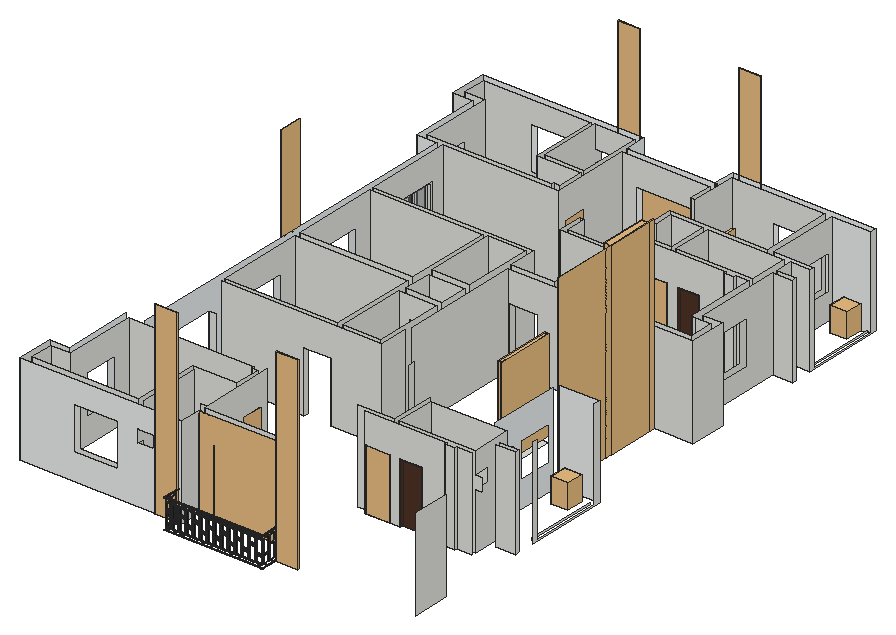
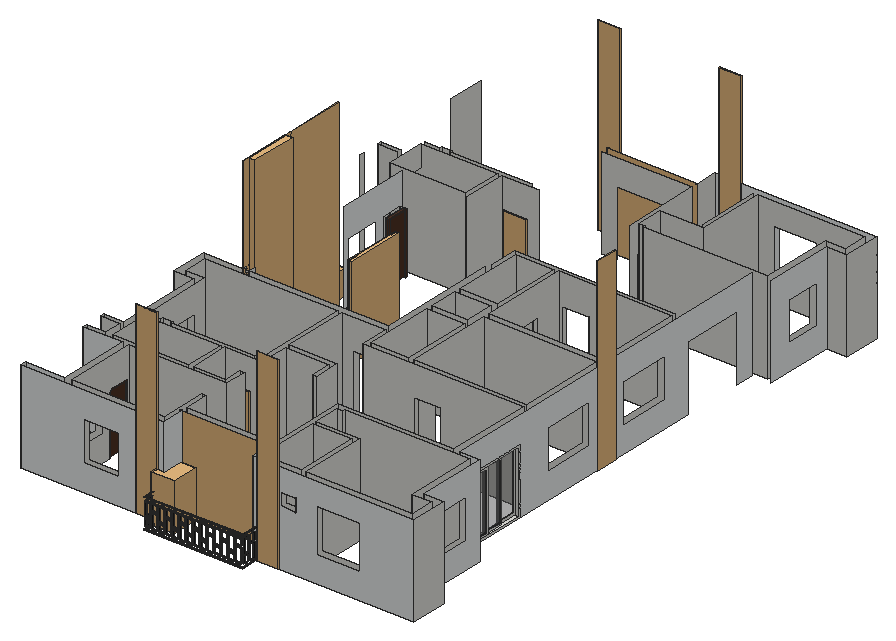
# SketchUp Ruby script. Lengths in inches.
U = 1.inch
M = Sketchup.active_model
def pt(a) = Geom::Point3d.new(a.map { |v| v * U })
def face(e, loops, mat)
  f = e.add_face(loops[0].map { |a| pt(a) })
  loops[1..].each { |l| e.add_face(l.map { |a| pt(a) }).erase! }
  f.material = f.back_material = mat if mat
  f
end
# faces: each face lists its corners as indices into pts; further lists are holes
def faces(e, pts, list, mat = nil) = list.each { |f| face(e, (f[0].is_a?(Array) ? f : [f]).map { |l| l.map { |i| pts[i] } }, mat) }
# xy, xz, yz: faces in a plane at the given z, y or x. An outline is a flat list of corners, or four numbers for a rectangle; further outlines are holes
def ring(l) = l.size == 4 ? [[l[0], l[1]], [l[2], l[1]], [l[2], l[3]], [l[0], l[3]]] : l.each_slice(2).to_a
def flat(e, list, mat, &to3) = list.each { |f| face(e, (f[0].is_a?(Array) ? f : [f]).map { |l| ring(l).map { |u, v| to3.(u, v) } }, mat) }
def xy(e, z, list, mat = nil) = flat(e, list, mat) { |x, y| [x, y, z] }
def xz(e, y, list, mat = nil) = flat(e, list, mat) { |x, z| [x, y, z] }
def yz(e, x, list, mat = nil) = flat(e, list, mat) { |y, z| [x, y, z] }
def lines(e, pts, list) = list.each { |a, b| e.add_line(pt(pts[a]), pt(pts[b])) }
# prism: a flat outline (further loops are holes) pulled along v
def prism(e, loops, v, mat = nil)
  f = face(e, loops, mat); d = Geom::Vector3d.new(v.map { |x| x * U })
  f.pushpull(f.normal.samedirection?(d) ? d.length : -d.length)
end
def box(e, o, s, mat = nil) = prism(e, [[o, [o[0] + s[0], o[1], o[2]], [o[0] + s[0], o[1] + s[1], o[2]], [o[0], o[1] + s[1], o[2]]]], [0, 0, s[2]], mat)
def at(x, y, z, deg = 0) = Geom::Transformation.translation(pt([x, y, z])) * Geom::Transformation.rotation(ORIGIN, Z_AXIS, deg.degrees)
def axes(o, x, y, z) = Geom::Transformation.new([*x, 0, *y, 0, *z, 0, *pt(o).to_a, 1])
def part(name) = M.definitions.add(name)
# library, detail: a bought-in or finely detailed component or shape, given as its bounding box
def library(name, o, s) = part(name).tap { |d| box(d.entities, o, s) }
def detail(e, o, s) = box(e.add_group.entities, o, s)
def put(e, d, t, mat = nil) = e.add_instance(d, t).tap { |i| i.material = mat if mat }
def group(e, t, mat = nil) = e.add_group.tap { |g| g.transformation = t; g.material = mat if mat }.entities
root = M.entities
M.materials.add("Polis06_194").color = [79, 50, 36]
M.materials.add("[3P0081_White-City]").color = [235, 238, 238]
M.materials.add("[Color M00]").color = [255, 255, 255]
M.materials.add("[Color M08]").color = [30, 30, 30]
M.materials.add("[Translucent Glass Gray]").color = [128, 128, 128]
M.materials["[Translucent Glass Gray]"].alpha = 0.5
c1 = part("구성 요소\#2")
prism(c1.entities,[[[0,0,0],[118.11,0,0],[118.11,0,78.74],[0,0,78.74]],[[116.14,0,76.77],[116.14,0,1.97],[1.97,0,1.97],[1.97,0,76.77]]],[0,7.875,0])
c2 = part("구성 요소\#1")
xy(c2.entities,0,[[[0,0,40.16,74.8],[2.375,2.375,37.78,72.43]]])
xy(c2.entities,1.18,[[2.375,2.375,37.78,72.43]],"[Translucent Glass Gray]")
xy(c2.entities,2.36,[[[0,0,40.16,74.8],[2.375,2.375,37.78,72.43]]])
xz(c2.entities,0,[[0,0,40.16,2.36]],"[Color M00]")
xz(c2.entities,2.375,[[2.375,0,37.78,1.18],[2.375,1.18,37.78,2.36]])
xz(c2.entities,72.43,[[2.375,0,37.78,1.18],[2.375,1.18,37.78,2.36]])
xz(c2.entities,74.8,[[0,0,40.16,2.36]],"[Color M00]")
yz(c2.entities,0,[[0,0,74.8,2.36]])
yz(c2.entities,2.375,[[2.375,0,72.43,1.18],[2.375,1.18,72.43,2.36]])
yz(c2.entities,37.78,[[2.375,0,72.43,1.18],[2.375,1.18,72.43,2.36]])
yz(c2.entities,40.16,[[0,0,74.8,2.36]])
c3 = part("구성 요소\#3")
xy(c3.entities,0,[[0,0,40.16,2.36]],"[Color M00]")
xy(c3.entities,2.375,[[2.375,0,37.78,1.18],[2.375,1.18,37.78,2.36]])
xy(c3.entities,35.83,[[38.48,0,39.47,0.39]])
xy(c3.entities,35.83,[[38.48,1.97,39.47,2.36]],"[Color M00]")
xy(c3.entities,38.98,[[38.48,0,39.47,0.39]])
xy(c3.entities,38.98,[[38.48,1.97,39.47,2.36]],"[Color M00]")
xy(c3.entities,72.43,[[2.375,0,37.78,1.18],[2.375,1.18,37.78,2.36]])
xy(c3.entities,74.8,[[0,0,40.16,2.36]],"[Color M00]")
xz(c3.entities,0,[[[0,0,40.16,74.8],[2.375,2.375,37.78,72.43],[38.48,35.83,39.47,38.98]]])
xz(c3.entities,0.39,[[38.48,35.83,39.47,38.98]])
xz(c3.entities,1.18,[[2.375,2.375,37.78,72.43]],"[Translucent Glass Gray]")
xz(c3.entities,1.97,[[38.48,35.83,39.47,38.98]],"[Color M00]")
xz(c3.entities,2.36,[[[0,0,40.16,74.8],[2.375,2.375,37.78,72.43],[38.48,35.83,39.47,38.98]]])
yz(c3.entities,0,[[0,0,2.36,74.8]])
yz(c3.entities,2.375,[[0,2.375,1.18,72.43],[1.18,2.375,2.36,72.43]])
yz(c3.entities,37.78,[[0,2.375,1.18,72.43],[1.18,2.375,2.36,72.43]])
yz(c3.entities,38.48,[[0,35.83,0.39,38.98]])
yz(c3.entities,38.48,[[1.97,35.83,2.36,38.98]],"[Color M00]")
yz(c3.entities,39.47,[[0,35.83,0.39,38.98]])
yz(c3.entities,39.47,[[1.97,35.83,2.36,38.98]],"[Color M00]")
yz(c3.entities,40.16,[[0,0,2.36,74.8]])
c4 = part("구성 요소\#4")
put(c4.entities,c2,axes([37.78,4.72,0],[1,0,0],[0,0,1],[0,-1,0]))
put(c4.entities,c3,at(75.5625,0,0))
put(c4.entities,c2,axes([0,7.09,0],[1,0,0],[0,0,1],[0,-1,0]))
c5 = part("그룹\#1")
put(c5.entities,c1,axes([0,0,0],[1.04,0,0],[0,1,0],[0,0,1]))
put(c5.entities,c4,axes([1.97,0.39,1.97],[1.02677,0,0],[0,1,0],[0,0,1]))
c6 = part("sliding door")
put(c6.entities,c5,at(0,0,0))
c7 = part("Flush door")
xy(c7.entities,0,[[0,0,4.72,1.18],[0,34.25,4.72,35.43]],"Polis06_194")
xy(c7.entities,85.26,[[0,1.18,4.72,34.25]],"Polis06_194")
xy(c7.entities,86.61,[[0,0,4.72,35.43]],"Polis06_194")
xz(c7.entities,0,[[0,0,4.72,86.61]],"Polis06_194")
xz(c7.entities,1.18,[[0,0,2.36,85.26],[2.36,0,4.72,85.26]],"Polis06_194")
xz(c7.entities,34.25,[[0,0,4.72,85.26]],"Polis06_194")
xz(c7.entities,35.43,[[0,0,4.72,86.61]],"Polis06_194")
yz(c7.entities,0,[[0,0,1.18,86.61],[34.25,0,35.43,86.61],[1.18,85.26,34.25,86.61]],"Polis06_194")
yz(c7.entities,2.36,[[1.18,0,34.25,0,34.25,85.21,1.18,85.26]],"Polis06_194")
yz(c7.entities,4.72,[[0,0,1.18,86.61],[34.25,0,35.43,86.61],[1.18,85.26,34.25,86.61]],"Polis06_194")
c8 = library("Plante 4",[-1.67,-6.5,0],[37.31,31.95,64.42])
c9 = library("Group\#241",[0,-0.25,0],[124.5,0.25,126])
c10 = library("19",[0,-1,0],[30,1,258])
c11 = library("Group\#100",[-9,0,0],[10,64,258])
c12 = library("Group\#105",[0,0,0],[0.75,82,258])
c13 = library("PINTU 6 YA",[0,-0.6875,0],[35.83,8.07,80.71])
c14 = library("Group\#2",[0,-3.15,0.41],[58,18.09,114.05])
c15 = part("Group\#70")
prism(c15.entities,[[[4.13,0,3.9375],[7.875,0,3.9375],[7.875,0,13.78],[4.13,0,13.78],[4.13,0,15.75],[7.875,0,15.75],[7.875,0,35.43],[4.13,0,35.43],[4.13,0,39.37],[3.74,0,39.37],[3.74,0,35.43],[0,0,35.43],[0,0,15.75],[3.74,0,15.75],[3.74,0,13.78],[0,0,13.78],[0,0,3.9375],[3.74,0,3.9375],[3.74,0,0],[4.13,0,0]],[[0.39,0,16.14],[0.39,0,35.04],[7.48,0,35.04],[7.48,0,16.14]],[[7.48,0,4.33],[0.39,0,4.33],[0.39,0,13.39],[7.48,0,13.39]]],[0,0.39,0],"[Color M08]")
c16 = part("Group\#69")
prism(c16.entities,[[[3.74,0,35.43],[0,0,35.43],[0,0,25.59],[3.74,0,25.59],[3.74,0,23.62],[0,0,23.62],[0,0,3.9375],[3.74,0,3.9375],[3.74,0,0],[4.13,0,0],[4.13,0,3.9375],[7.875,0,3.9375],[7.875,0,23.62],[4.13,0,23.62],[4.13,0,25.59],[7.875,0,25.59],[7.875,0,35.43],[4.13,0,35.43],[4.13,0,39.37],[3.74,0,39.37]],[[7.48,0,23.23],[7.48,0,4.33],[0.39,0,4.33],[0.39,0,23.23]],[[0.39,0,35.04],[7.48,0,35.04],[7.48,0,25.98],[0.39,0,25.98]]],[0,0.39,0],"[Color M08]")
c17 = part("Group\#71")
put(c17.entities,c15,at(0,0,0))
put(c17.entities,c16,at(9.84,0,0))
c18 = part("Group\#81")
g1 = group(c18.entities,at(0,0,0))
prism(g1,[[[24,-19.7,0],[0,-19.7,0],[0,120.08,0],[24,120.08,0],[24,118.11,0],[1.97,118.11,0],[1.97,-17.76,0],[24,-17.76,0]]],[0,0,0.79],"[Color M08]")
put(c18.entities,c17,axes([0.79,40.35,0.79],[0,1,0],[1,0,0],[0,0,1]))
put(c18.entities,c17,at(2.95,118.9,0.79))
put(c18.entities,c17,axes([0.79,79.72,0.79],[0,1,0],[1,0,0],[0,0,1]))
put(c18.entities,c17,axes([0.79,60.04,0.79],[0,1,0],[1,0,0],[0,0,1]))
put(c18.entities,c17,axes([0.79,99.41,0.79],[0,1,0],[1,0,0],[0,0,1]))
put(c18.entities,c17,axes([0.79,0.98,0.79],[0,1,0],[1,0,0],[0,0,1]))
g2 = group(c18.entities,at(0,0,40.16))
prism(g2,[[[24,-19.7,0],[0,-19.7,0],[0,120.08,0],[24,120.08,0],[24,118.11,0],[1.97,118.11,0],[1.97,-17.76,0],[24,-17.76,0]]],[0,0,0.79],"[Color M08]")
put(c18.entities,c17,axes([0.79,20.67,0.79],[0,1,0],[1,0,0],[0,0,1]))
put(c18.entities,c17,axes([0.79,-18.7,0.79],[0,1,0],[1,0,0],[0,0,1]))
put(c18.entities,c17,axes([2.95,-18.49,0.79],[1,0,0],[0,-1,0],[0,0,1]))
c19 = library("Gruppo\#3",[0,0,0],[23.62,24.19,33.46])
c20 = library("Group\#126",[0,0,0],[0.75,82,258])
xy(root,132,[[308,361.97,325.5,362.97],[198,614.97,198,656.97,207,656.97,207,630.97,321,630.97,321,624.97,207,624.97,207,614.97],[198,656.97,202,724.97],[202,656.97,203,724.97],[203,656.97,207,724.97],
  [553.5,675.97,562.5,741.97],[198,724.97,207,726.97],[384.75,779.97,402.25,783.97],[198,785.97,202,853.97],[202,785.97,203,853.97],
  [203,785.97,207,853.97],[171,1029.97,180,1031.97]])
xz(root,357.97,[[[144,132,366,258],[218,168,278,228],[306,210,327.5,228]]],"[3P0081_White-City]")
xz(root,366.97,[[[153,132,300,258],[218,168,278,228]]])
xz(root,387.97,[[366,132,386.25,132,386.25,222,470.25,222,470.25,132,490.5,132,490.5,258,366,258]],"[3P0081_White-City]")
xz(root,396.97,[[366,132,366,258,490.5,258,490.5,132,470.25,132,470.25,222,386.25,222,386.25,132]])
xz(root,399.97,[[153,132,180,258]])
xz(root,408.97,[[144,132,171,258]])
xz(root,459.97,[[300,132,300,258,360,258,360,132,333,132,333,216,309,216,309,132]])
xz(root,462.97,[[360,132,366,216]])
xz(root,495.97,[[352,132,360,258],[617.5,132,631.5,258]])
xz(root,498.97,[[180,132,352,258],[504.5,132,507,132,507,216,539,216,539,132,553.5,132,553.5,216,583.5,216,583.5,132,617.5,132,617.5,258,504.5,258],[631.5,132,652.5,258]])
xz(root,504.97,[[490.5,132,490.5,258,541.5,258,541.5,132,539,132,539,216,507,216,507,132],[547.5,132,547.5,258,652.5,258,652.5,228,661.5,228,661.5,210,652.5,210,652.5,132,583.5,132,583.5,216,553.5,216,553.5,132]])
xz(root,529,[[661.5,132,688.5,258]])
xz(root,535,[[661.5,132,688.5,258]])
xz(root,558.97,[[547.5,132,652.5,258]])
xz(root,567.97,[[622.5,132,631.5,216]])
xz(root,614.97,[[198,132,207,222]])
xz(root,624.97,[[207,132,321,132,321,216,357,216,357,132,427.5,132,427.5,258,207,258]])
xz(root,630.97,[[207,132,207,258,363,258,363,132,357,132,357,216,321,216,321,132],[369,132,421.5,258]])
xz(root,666.97,[[363,132,369,216]])
xz(root,672.97,[[631.5,132,688.5,258]],"[3P0081_White-City]")
xz(root,726.97,[[[369,132,421.5,258],[382.75,210,404.25,228]]])
xz(root,735.97,[[[372,132,421.5,258],[382.75,210,404.25,228]]])
xz(root,750.97,[[207,132,363,258]])
xz(root,759.97,[[207,132,363,258]])
xz(root,774.97,[[[372,132,421.5,258],[382.75,210,404.25,228]]])
xz(root,783.97,[[[369,132,421.5,258],[382.75,210,404.25,228]]])
xz(root,827.97,[[622.5,132,631.5,258]])
xz(root,837.97,[[430.5,132,433.5,132,433.5,216,472.5,216,472.5,132,622.5,132,622.5,258,430.5,258],[631.5,132,685.5,258]])
xz(root,846.97,[[427.5,132,427.5,258,487.5,258,487.5,132,472.5,132,472.5,216,433.5,216,433.5,132],[493.5,132,676.5,258]])
xz(root,879.97,[[207,132,321,132,321,216,357,216,357,132,363,132,363,258,207,258],[369,132,421.5,258],[649.5,132,654.5,258],[654.5,132,676.5,258]])
xz(root,885.97,[[207,132,207,258,427.5,258,427.5,132,357,132,357,216,321,216,321,132]])
xz(root,888.97,[[658.5,132,685.5,258]])
xz(root,938.47,[[421.5,132,487.5,258]])
xz(root,944.47,[[427.5,132,487.5,258]])
xz(root,972.97,[[421.5,132,427.5,258]])
xz(root,975.97,[[493.5,132,501.5,258],[617.5,132,631.5,258]])
xz(root,978.97,[[501.5,132,504,132,504,216,536,216,536,132,550.5,132,550.5,216,580.5,216,580.5,132,617.5,132,617.5,258,501.5,258],[631.5,132,649.5,258]])
xz(root,984.97,[[487.5,132,487.5,258,538.5,258,538.5,132,536,132,536,216,504,216,504,132],[544.5,132,544.5,258,649.5,258,649.5,132,580.5,132,580.5,216,550.5,216,550.5,132]])
xz(root,987.97,[[198,132,207,222]])
xz(root,1005.97,[[207,132,366,258]])
xz(root,1005.97,[[171,132,198,258]],"[3P0081_White-City]")
xz(root,1009,[[658.5,132,685.5,258]])
xz(root,1011.97,[[180,132,352,258]])
xz(root,1014.97,[[352,132,360,258],[487.5,132,493.5,258]])
xz(root,1015,[[658.5,132,685.5,258]])
xz(root,1017.47,[[360,132,366,216]])
xz(root,1038.97,[[493.5,132,538.5,258],[544.5,132,649.5,132,649.5,210,658.5,210,658.5,132,685.5,132,685.5,258,658.5,258,658.5,228,649.5,228,649.5,258,544.5,258]])
xz(root,1044.97,[[487.5,132,622.5,258]])
xz(root,1044.97,[[631.5,132,631.5,258,685.5,258,685.5,134,679.5,134,679.5,132]],"[3P0081_White-City]")
xz(root,1050.97,[[300,132,309,132,309,216,333,216,333,132,360,132,360,258,300,258]])
xz(root,1056.97,[[306,132,306,258,360,258,360,132,333,132,333,216,309,216,309,132]])
xz(root,1080.97,[[487.5,132,513.5,132,513.5,168,493.5,168,493.5,258,487.5,258]])
xz(root,1086.97,[[493.5,132,513.5,168]])
xz(root,1101.97,[[144,132,171,258]])
xz(root,1110.97,[[153,132,180,258]])
xz(root,1113.97,[[366,132,386.25,132,386.25,222,470.25,222,470.25,132,487.5,132,487.5,258,366,258]])
xz(root,1122.97,[[366,132,366,258,487.5,258,487.5,132,470.25,132,470.25,222,386.25,222,386.25,132]],"[3P0081_White-City]")
xz(root,1143.97,[[[153,132,300,258],[218,168,278,228]],[306,132,360,132,360,258,306,258,306,228,327.5,228,327.5,210,306,210],[[493.5,132,622.5,258],[550.5,168,598.5,222]]])
xz(root,1143.97,[[631.5,132,679.5,132,679.5,134,685.5,134,685.5,258,631.5,258]],"[3P0081_White-City]")
xz(root,1152.97,[[[144,132,366,258],[218,168,278,228],[306,210,327.5,228]],[[487.5,132,685.5,258],[550.5,168,598.5,222]]],"[3P0081_White-City]")
yz(root,144,[[357.97,132,408.97,258],[1101.97,132,1152.97,258]])
yz(root,153,[[366.97,132,399.97,258],[1110.97,132,1143.97,258]])
yz(root,171,[[[408.97,132,504.97,258],[426.87,168,474.87,222]],[[1005.97,132,1101.97,258],[1029.97,168,1077.97,222]]],"[3P0081_White-City]")
yz(root,180,[[[399.97,132,498.97,258],[426.87,168,474.87,222]],[[1011.97,132,1110.97,258],[1029.97,168,1077.97,222]]])
yz(root,198,[[[504.97,132,504.97,258,1005.97,258,1005.97,132,987.97,132,987.97,222,903.97,222,903.97,132,614.97,132,614.97,222,530.97,222,530.97,132],[654.97,168,726.97,222],[783.97,168,855.97,222]]],"[3P0081_White-City]")
yz(root,207,[[[630.97,132,750.97,258],[654.97,168,726.97,222]],[[759.97,132,879.97,258],[783.97,168,855.97,222]],[885.97,132,903.97,132,903.97,222,987.97,222,987.97,132,1005.97,132,1005.97,258,885.97,258]])
yz(root,300,[[366.97,132,459.97,258],[1050.97,132,1143.97,258]])
yz(root,306,[[366.97,132,453.97,132,453.97,258,366.97,258,366.97,228,357.97,228,357.97,210,366.97,210],[1056.97,132,1143.97,132,1143.97,210,1152.97,210,1152.97,228,1143.97,228,1143.97,258,1056.97,258]])
yz(root,309,[[1050.97,132,1056.97,216]])
yz(root,321,[[624.97,132,630.97,216]])
yz(root,333,[[1050.97,132,1056.97,216]])
yz(root,352,[[495.97,132,498.97,258],[1011.97,132,1014.97,258]])
yz(root,357,[[624.97,132,630.97,216],[879.97,132,885.97,216]])
yz(root,360,[[459.97,132,459.97,258,495.97,258,495.97,132,492.97,132,492.97,216,462.97,216,462.97,132],[1014.97,132,1014.97,258,1050.97,258,1050.97,132,1047.47,132,1047.47,216,1017.47,216,1017.47,132],[1056.97,132,1143.97,258]])
yz(root,363,[[630.97,132,630.97,258,750.97,258,750.97,132,690.97,132,690.97,216,666.97,216,666.97,132],[759.97,132,759.97,258,879.97,258,879.97,132,843.97,132,843.97,216,819.97,216,819.97,132]])
yz(root,366,[[357.97,132,387.97,258],[396.97,132,462.97,132,462.97,216,492.97,216,492.97,132,504.97,132,504.97,258,396.97,258],[1005.97,132,1017.47,132,1017.47,216,1047.47,216,1047.47,132,1113.97,132,1113.97,258,1005.97,258]])
yz(root,366,[[1122.97,132,1152.97,258]],"[3P0081_White-City]")
yz(root,369,[[630.97,132,666.97,132,666.97,216,690.97,216,690.97,132,726.97,132,726.97,258,630.97,258],[783.97,132,819.97,132,819.97,216,843.97,216,843.97,132,879.97,132,879.97,258,783.97,258]])
yz(root,372,[[735.97,132,774.97,258]])
yz(root,386.25,[[387.97,132,396.97,222]])
yz(root,421.5,[[630.97,132,726.97,258],[735.97,132,774.97,258],[783.97,132,879.97,258],[938.47,132,972.97,258]])
yz(root,427.5,[[624.97,132,663.97,258],[846.97,132,885.97,258],[944.47,132,972.97,258]])
yz(root,430.5,[[672.97,132,837.97,258]])
yz(root,433.5,[[663.97,132,672.97,216],[837.97,132,846.97,216]])
yz(root,487.5,[[846.97,132,938.47,258],[944.47,132,984.97,258],[1014.97,132,1044.97,258],[1080.97,132,1113.97,258]])
yz(root,487.5,[[1122.97,132,1152.97,258]],"[3P0081_White-City]")
yz(root,493.5,[[846.97,132,975.97,258],[1014.97,132,1038.97,258],[1086.97,132,1143.97,132,1143.97,258,1080.97,258,1080.97,168,1086.97,168]])
yz(root,501.5,[[975.97,132,978.97,258]])
yz(root,538.5,[[984.97,132,1038.97,258]])
yz(root,539,[[498.97,132,504.97,216]])
yz(root,541.5,[[504.97,132,564.97,258]])
yz(root,544.5,[[984.97,132,1038.97,258]])
yz(root,547.5,[[504.97,132,558.97,258]])
yz(root,553.5,[[498.97,132,504.97,216],[672.97,132,672.97,258,678.97,258,678.97,134,738.97,134,738.97,258,753.97,258,753.97,132]])
yz(root,580.5,[[978.97,132,984.97,216]])
yz(root,617.5,[[495.97,132,498.97,258],[975.97,132,978.97,258]])
yz(root,622.5,[[827.97,132,837.97,258],[[1044.97,132,1044.97,258,1143.97,258,1143.97,132,1077.97,132,1077.97,216,1047.97,216,1047.97,132],[1089.97,168,1137.97,216]]])
yz(root,631.5,[[495.97,132,498.97,258],[827.97,132,837.97,258],[975.97,132,978.97,258],[[1044.97,132,1047.97,132,1047.97,216,1077.97,216,1077.97,132,1143.97,132,1143.97,258,1044.97,258],[1089.97,168,1137.97,216]]])
yz(root,631.5,[[[564.97,132,567.97,132,567.97,216,597.97,216,597.97,132,663.97,132,663.97,258,564.97,258],[609.97,168,657.97,216]]],"[3P0081_White-City]")
yz(root,649.5,[[[879.97,132,978.97,258],[897.97,162,963.97,222]],[984.97,132,984.97,258,1038.97,258,1038.97,228,1017.47,228,1017.47,210,1038.97,210,1038.97,132]])
yz(root,652.5,[[504.97,132,504.97,210,526.53,210,526.53,228,504.97,228,504.97,258,558.97,258,558.97,132]])
yz(root,658.5,[[[888.97,132,1009,258],[897.97,162,963.97,222]],[1015,132,1038.97,132,1038.97,210,1017.47,210,1017.47,228,1038.97,228,1038.97,258,1015,258]])
yz(root,676.5,[[846.97,132,879.97,258]])
yz(root,679.5,[[1044.97,132,1143.97,134]])
yz(root,682.5,[[564.97,132,663.97,134]])
yz(root,685.5,[[837.97,132,888.97,258],[1009,132,1015,258],[1038.97,132,1152.97,132,1152.97,258,1143.97,258,1143.97,134,1044.97,134,1044.97,258,1038.97,258]])
yz(root,688.5,[[357.97,132,408.97,258],[529,132,535,258],[558.97,132,672.97,132,672.97,258,663.97,258,663.97,134,564.97,134,564.97,258,558.97,258]])
put(root,c6,axes([198,903.97,132],[0,0.68385,0],[1,0,0],[0,0,1.143]))
put(root,c7,axes([627.22,597.97,132],[-1,0,0],[0,-0.84667,0],[0,0,0.96982]))
put(root,c7,axes([627.22,1077.97,132],[-1,0,0],[0,-0.84667,0],[0,0,0.96982]))
put(root,c8,at(491.29,1126.79,132,90))
put(root,c9,at(366,387.97,132))
put(root,c9,axes([366,1122.97,132],[1,0,0],[0,-1,0],[0,0,1]))
put(root,c10,at(330,357.97,132))
put(root,c10,axes([526.5,357.97,132],[-1,0,0],[0,1,0],[0,0,1]))
put(root,c10,axes([330,1152.97,132],[1,0,0],[0,-1,0],[0,0,1]))
put(root,c10,at(526.5,1152.97,132,180))
put(root,c10,axes([198,740.47,132],[0,1,0],[1,0,0],[0,0,1]))
put(root,c11,at(631.5,763.97,132))
put(root,c12,at(631.5,672.97,132))
put(root,c13,axes([539,499.66,132],[-0.89311,0,0],[0,1,0],[0,0,1.04078]))
put(root,c13,axes([536,979.66,132],[-0.89311,0,0],[0,1,0],[0,0,1.04078]))
put(root,c13,axes([365.3125,462.99,132],[0.01802,0.8369,0],[-0.99977,0.02153,0],[0,0,1.04078]))
put(root,c13,axes([365.3125,1047.96,132],[0.01802,-0.8369,0],[-0.99977,-0.02153,0],[0,0,1.04078]))
put(root,c14,axes([549.76,753.97,131.54],[0,-1.39655,0],[0.34,0,0],[0,0,1.10484]))
put(root,c18,axes([477.26,333.97,132],[0,1,0],[-0.97654,0,0],[0,0,1]))
put(root,c18,axes([477.26,1176.97,132],[0,-1,0],[-0.97654,0,0],[0,0,1]))
put(root,c19,at(647.91,639.78,132))
put(root,c19,at(647.91,1119.78,132))
put(root,c20,at(631.5,754.98,132))
put(root,c7,axes([583.5,504.39,132],[0,-1,0],[-0.84667,0,0],[0,0,0.96982]))
put(root,c7,axes([580.5,984.39,132],[0,-1,0],[-0.84667,0,0],[0,0,0.96982]))
